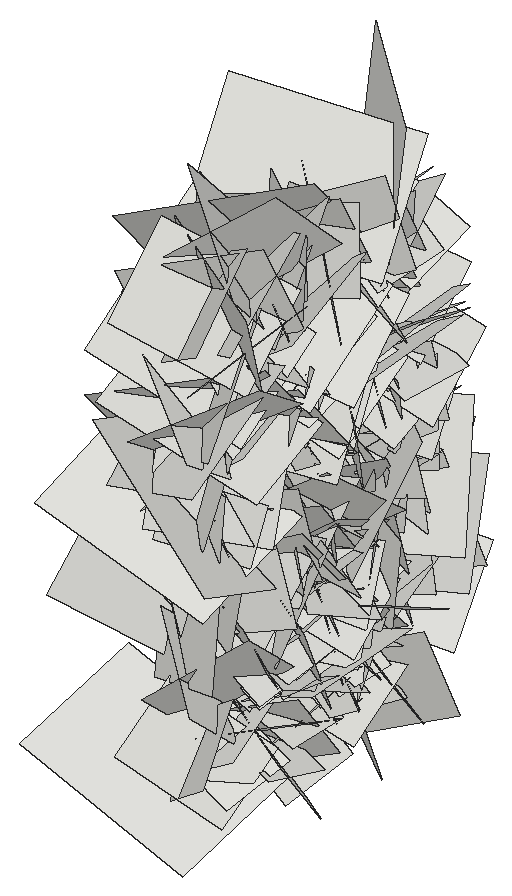
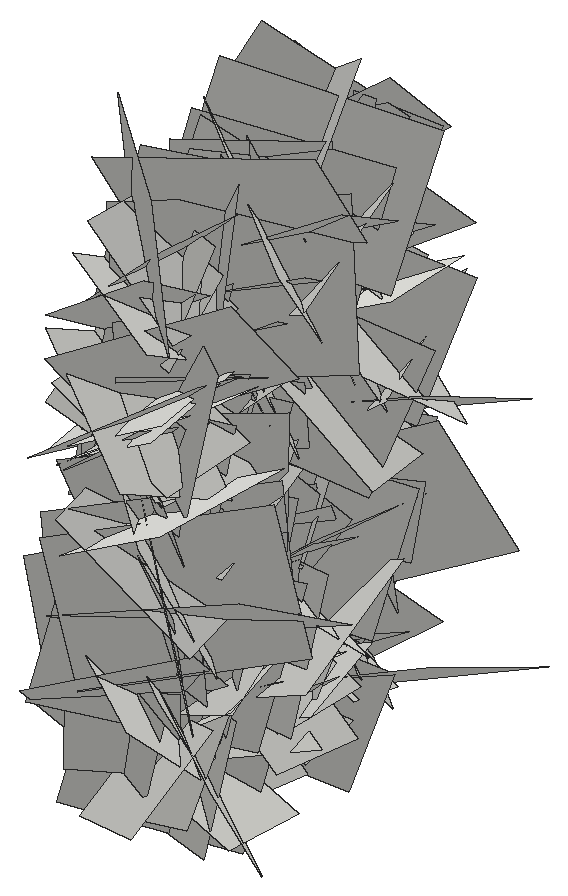
# SketchUp Ruby script. Lengths in inches.
U = 1.inch
M = Sketchup.active_model
def pt(a) = Geom::Point3d.new(a.map { |v| v * U })
def face(e, loops, mat)
  f = e.add_face(loops[0].map { |a| pt(a) })
  loops[1..].each { |l| e.add_face(l.map { |a| pt(a) }).erase! }
  f.material = f.back_material = mat if mat
  f
end
# faces: each face lists its corners as indices into pts; further lists are holes
def faces(e, pts, list, mat = nil) = list.each { |f| face(e, (f[0].is_a?(Array) ? f : [f]).map { |l| l.map { |i| pts[i] } }, mat) }
# xy, xz, yz: faces in a plane at the given z, y or x. An outline is a flat list of corners, or four numbers for a rectangle; further outlines are holes
def ring(l) = l.size == 4 ? [[l[0], l[1]], [l[2], l[1]], [l[2], l[3]], [l[0], l[3]]] : l.each_slice(2).to_a
def flat(e, list, mat, &to3) = list.each { |f| face(e, (f[0].is_a?(Array) ? f : [f]).map { |l| ring(l).map { |u, v| to3.(u, v) } }, mat) }
def xy(e, z, list, mat = nil) = flat(e, list, mat) { |x, y| [x, y, z] }
def xz(e, y, list, mat = nil) = flat(e, list, mat) { |x, z| [x, y, z] }
def yz(e, x, list, mat = nil) = flat(e, list, mat) { |y, z| [x, y, z] }
def lines(e, pts, list) = list.each { |a, b| e.add_line(pt(pts[a]), pt(pts[b])) }
# prism: a flat outline (further loops are holes) pulled along v
def prism(e, loops, v, mat = nil)
  f = face(e, loops, mat); d = Geom::Vector3d.new(v.map { |x| x * U })
  f.pushpull(f.normal.samedirection?(d) ? d.length : -d.length)
end
def box(e, o, s, mat = nil) = prism(e, [[o, [o[0] + s[0], o[1], o[2]], [o[0] + s[0], o[1] + s[1], o[2]], [o[0], o[1] + s[1], o[2]]]], [0, 0, s[2]], mat)
def at(x, y, z, deg = 0) = Geom::Transformation.translation(pt([x, y, z])) * Geom::Transformation.rotation(ORIGIN, Z_AXIS, deg.degrees)
def axes(o, x, y, z) = Geom::Transformation.new([*x, 0, *y, 0, *z, 0, *pt(o).to_a, 1])
def part(name) = M.definitions.add(name)
# library, detail: a bought-in or finely detailed component or shape, given as its bounding box
def library(name, o, s) = part(name).tap { |d| box(d.entities, o, s) }
def detail(e, o, s) = box(e.add_group.entities, o, s)
def put(e, d, t, mat = nil) = e.add_instance(d, t).tap { |i| i.material = mat if mat }
def group(e, t, mat = nil) = e.add_group.tap { |g| g.transformation = t; g.material = mat if mat }.entities
root = M.entities
c1 = part("Component\#6")
p = [[0.01,0,0],[0,3.24,4.54],[4.32,3.24,4.54],[4.33,0,0]]
faces(c1.entities,p,[[0,1,2,3]])
put(root,c1,axes([18.5,161.87,9.58],[-0.35888,-0.49511,-1.17449],[-0.11741,-1.19919,0.53746],[-1.34594,0.23663,0.26628]))
put(root,c1,axes([18.5,170.67,8.29],[-0.13658,-1.14766,-0.62909],[-0.33753,-0.58565,1.13362],[-1.34561,0.26339,-0.2205]))
put(root,c1,axes([18.5,160.65,1.35],[-0.1594,-1.22011,-0.46707],[-0.28659,-0.43091,1.2127],[-1.35486,0.2347,-0.20157]))
put(root,c1,axes([18.5,161.24,11.55],[-0.08722,-1.18104,-0.51149],[-0.30261,-0.48302,1.16122],[-1.33028,0.18731,-0.23062]))
put(root,c1,axes([18.5,161.91,24.73],[-0.20116,0.87735,-0.9177],[-0.06395,-0.93308,-0.87958],[-1.34427,-0.0869,0.17917]))
put(root,c1,axes([18.5,167.61,21.95],[-0.32344,0.31012,-1.26322],[0.1451,-1.28265,-0.34796],[-1.37111,-0.2089,0.26116]))
put(root,c1,axes([18.5,171.01,11.29],[-0.23144,-0.15428,-1.27652],[0.01824,-1.29503,0.15357],[-1.36284,0.00887,0.21884]))
put(root,c1,axes([18.5,161.07,7.88],[-0.0926,0.91308,0.78861],[-0.24837,0.76278,-0.90913],[-1.25453,-0.21841,0.12178]))
put(root,c1,axes([18.5,170.58,10.37],[-0.24309,-1.14649,0.14454],[-0.04952,0.15643,1.16674],[-1.2239,0.22139,-0.07591]))
put(root,c1,axes([18.5,165.1,2.71],[0.06092,-1.21711,0.58199],[-0.18306,0.57109,1.21136],[-1.41828,-0.12599,-0.13136]))
put(root,c1,axes([18.5,162.31,11.53],[-0.17206,0.75955,-0.87532],[-0.12131,-0.89005,-0.75111],[-1.22246,-0.01858,0.19774]))
put(root,c1,axes([18.5,157.93,15.34],[-0.27083,1.19165,0.15594],[0.0802,0.17506,-1.21378],[-1.27139,-0.2428,-0.10978]))
put(root,c1,axes([18.5,168.375,23.9],[0.0952,-0.72561,-1.04974],[-0.29336,-1.03837,0.69407],[-1.32049,0.17837,-0.22987]))
put(root,c1,axes([18.5,159.14,18.38],[-0.07521,0.79304,-0.86536],[-0.12573,-0.86735,-0.78513],[-1.23784,0.03991,0.13233]))
put(root,c1,axes([18.5,155.03,14.95],[0.10989,1.07322,0.82249],[-0.07177,0.82799,-1.07186],[-1.43147,0.04087,0.11688]))
put(root,c1,axes([18.5,166.4,18.65],[0.092,-1.19571,-0.63762],[-0.0325,-0.6405,1.19693],[-1.43603,-0.06211,-0.06794]))
put(root,c1,axes([18.5,159.69,18.96],[-0.02704,0.74145,1.09535],[0.09362,1.09406,-0.73853],[-1.39894,0.05888,-0.07059]))
put(root,c1,axes([18.5,163.36,23.49],[-0.04873,0.57368,-1.00395],[-0.12423,-1.00188,-0.56714],[-1.21936,0.07915,0.09791]))
put(root,c1,axes([18.5,162.85,15.75],[-0.04254,-1.00522,0.67204],[-0.02385,0.67292,1.00519],[-1.28151,0.02084,-0.04102]))
put(root,c1,axes([18.5,163.86,1.73],[-0.03729,0.66749,1.03354],[0.00972,1.03407,-0.66752],[-1.30413,-0.01138,-0.03452]))
put(root,c1,axes([18.5,161.03,16.77],[0.02327,0.73455,-0.90907],[-0.17416,-0.89826,-0.72978],[-1.22657,0.14148,0.08637]))
put(root,c1,axes([18.5,162.03,18.62],[-0.15865,-0.78055,-0.79386],[0.03617,-0.80384,0.78393],[-1.17956,0.08034,0.13081]))
put(root,c1,axes([18.5,161.02,12.77],[-0.04866,0.36936,-1.04237],[-0.12613,-1.03886,-0.36288],[-1.16543,0.09701,0.0828]))
put(root,c1,axes([18.5,163.21,2.24],[0.08398,-0.53221,1.10764],[-0.11648,1.10243,0.53756],[-1.29738,-0.13342,0.02343]))
put(root,c1,axes([18.5,155.93,16.01],[-0.06166,0.77521,1.08886],[0.24821,1.07895,-0.75564],[-1.39492,0.15772,-0.18259]))
put(root,c1,axes([14.53,164.09,3.1],[-0.16189,-0.51758,0.36968],[-0.06161,0.38995,0.52196],[0.67139,-0.08902,0.13704]))
put(root,c1,axes([18.5,165.97,13.03],[-0.11695,-0.23373,1.15092],[0.10796,1.14973,0.24325],[-1.24018,0.12213,-0.08736]))
put(root,c1,axes([18.5,170.79,17.67],[-0.07972,-0.69903,-0.88266],[0.01234,-0.88506,0.69994],[-1.19343,0.03754,0.0662]))
put(root,c1,axes([18.5,164.53,2.65],[-0.11418,0.95876,0.15487],[-0.16789,0.13639,-0.95453],[-1.01568,-0.13033,0.14037]))
put(root,c1,axes([18.5,165.6875,8.33],[-0.14254,-0.77018,0.64298],[-0.05856,0.65343,0.77114],[-1.06187,0.06735,-0.12884]))
put(root,c1,axes([14.53,159.77,13.93],[-0.14822,0.47929,0.38572],[0.01533,0.39801,-0.48932],[0.65196,0.0996,0.0992]))
put(root,c1,axes([18.5,164.18,5.53],[-0.00871,-1.21515,-0.1589],[0.11926,-0.15898,1.20995],[-1.29354,-0.00648,0.11262]))
put(root,c1,axes([18.5,168.99,0.33],[-0.20008,-0.71049,0.66963],[0.07161,0.67089,0.73087],[-1.03242,0.18422,-0.07908]))
put(root,c1,axes([18.5,166.625,12.7],[-0.17127,1.04033,-0.10676],[0.13463,-0.08771,-1.04688],[-1.10034,-0.17266,-0.11147]))
put(root,c1,axes([18.5,160.14,4.78],[-0.03826,-0.47304,0.81506],[-0.18962,0.80427,0.45886],[-0.98077,-0.13704,-0.12051]))
put(root,c1,axes([14.53,170.02,6.34],[-0.13634,-0.30577,-0.6303],[-0.02329,-0.63876,0.31436],[0.74222,-0.07621,-0.10592]))
put(root,c1,axes([18.5,156.14,6.5],[-0.17845,0.35117,0.84391],[-0.01887,0.85668,-0.36003],[-0.96872,-0.08137,-0.14844]))
put(root,c1,axes([18.5,163.93,5.47],[-0.11462,-1.01834,-0.26907],[0.10191,-0.2789,1.0169],[-1.11183,0.07941,0.12095]))
put(root,c1,axes([14.53,162.91,7.6875],[-0.03517,0.6334,0.29771],[-0.1292,0.28826,-0.62688],[0.73053,0.08147,-0.09654]))
put(root,c1,axes([18.5,160.62,5.12],[-0.08568,1.04485,0.18773],[0.09569,0.19436,-1.04286],[-1.1212,-0.06325,-0.10335]))
put(root,c1,axes([18.5,162.44,14.8125],[0.22172,-1.13603,-0.19278],[-0.19013,-0.22565,1.13507],[-1.20652,-0.17321,-0.21429]))
put(root,c1,axes([18.5,159.91,9.22],[0.2022,-1.20502,0.50539],[0.1049,0.52261,1.20871],[-1.38114,-0.13672,0.1658]))
put(root,c1,axes([18.5,163.57,3.71],[-0.11292,-0.2033,0.99476],[0.09749,0.99417,0.21302],[-1.07181,0.11185,-0.08542]))
put(root,c1,axes([18.5,166.01,11.8],[-0.21466,0.53877,-0.68228],[0.03009,-0.69607,-0.55809],[-0.92102,-0.14831,0.14079]))
put(root,c1,axes([18.5,168.87,14.79],[-0.03205,0.06087,-1.12787],[0.16204,-1.11767,-0.06442],[-1.18627,-0.15431,0.02167]))
put(root,c1,axes([18.5,167.18,1.59],[0.07507,-1.0991,0.32301],[0.05871,0.32653,1.09895],[-1.2129,-0.05222,0.07319]))
put(root,c1,axes([18.5,157.18,19.73],[0.07599,0.81527,0.8297],[0.084,0.82592,-0.8184],[-1.23014,0.10676,-0.00463]))
put(root,c1,axes([18.5,167.28,17.92],[0.19972,-0.96368,-0.57877],[-0.14667,-0.60226,0.95775],[-1.18251,-0.08806,-0.21655]))
put(root,c1,axes([18.5,167.22,15.375],[0.0235,-0.92066,-0.53568],[0.01768,-0.53543,0.92093],[-1.12894,-0.02755,0.00327]))
put(root,c1,axes([14.53,162.79,15.86],[-0.07285,0.46729,0.4905],[0.02436,0.49435,-0.46773],[0.71769,0.03066,0.06566]))
put(root,c1,axes([14.53,161.25,17.66],[-0.25985,0.898,-0.37026],[-0.14737,-0.41038,-0.90325],[1.01902,0.16964,-0.22504]))
put(root,c1,axes([14.53,165.96,10.85],[-0.09912,0.20412,-0.70693],[-0.02587,-0.71308,-0.20267],[0.77953,0.00229,-0.09661]))
put(root,c1,axes([18.5,169.19,10.7],[0.0913,0.46499,-1.24639],[0.29576,-1.22753,-0.43867],[-1.37875,-0.23253,-0.17663]))
put(root,c1,axes([18.5,168.14,0.12],[0.06773,-0.63363,0.78179],[-0.11595,0.77435,0.63654],[-1.06038,-0.12515,-0.01967]))
put(root,c1,axes([18.5,166.18,19.56],[0.12535,0.0531,1.28965],[0.2192,1.27754,-0.07157],[-1.35051,0.21229,0.10808]))
put(root,c1,axes([18.5,167.01,8.33],[-0.18631,0.3359,0.73427],[-0.04897,0.74605,-0.35235],[-0.8545,-0.11599,-0.1399]))
put(root,c1,axes([14.53,159.82,10.86],[-0.164,0.05549,-0.7166],[0.119,-0.72215,-0.08015],[0.75252,0.12629,-0.14349]))
put(root,c1,axes([18.5,164.72,6.23],[0.02586,0.29335,1.1723],[0.23754,1.1511,-0.29271],[-1.25874,0.22326,-0.03115]))
put(root,c1,axes([14.53,164.71,11.17],[-0.09162,-0.23701,0.75882],[-0.09076,0.76162,0.22813],[0.83777,0.05659,0.1077]))
put(root,c1,axes([14.53,167.39,12.19],[-0.06725,0.11282,-0.6237],[0.12717,-0.61335,-0.12315],[0.65971,0.12973,-0.03984]))
put(root,c1,axes([14.53,158.25,7.85],[0.01053,0.60228,-0.51533],[-0.19634,-0.49934,-0.58716],[0.81696,-0.12777,-0.13447]))
put(root,c1,axes([18.5,165.51,17.74],[-0.00528,-0.97827,-0.44464],[0.11526,-0.44282,0.97306],[-1.13321,-0.04048,0.10104]))
put(root,c1,axes([18.5,165.75,-1.09],[0.03685,-0.4153,0.96157],[0.02645,0.96216,0.41465],[-1.10996,0.00914,0.04181]))
put(root,c1,axes([18.5,167.74,3.51],[0.11337,-0.86322,0.3774],[-0.28126,0.33685,0.84566],[-0.95821,-0.201,-0.20357]))
put(root,c1,axes([18.5,161.03,4.22],[-0.00206,0.54706,-0.73945],[-0.10036,-0.73565,-0.544],[-0.96983,0.07497,0.05787]))
put(root,c1,axes([18.5,158.84,13.7],[-0.15038,-0.75335,0.50607],[0.08727,0.49942,0.76653],[-0.95804,0.16374,-0.00961]))
put(root,c1,axes([18.5,166.72,20.27],[-0.14718,0.45385,-0.66356],[-0.05291,-0.67695,-0.45256],[-0.85051,-0.03642,0.14299]))
put(root,c1,axes([14.53,158.82,19.64],[0.09205,0.73549,-0.019],[-0.17536,0.00088,-0.72213],[0.75991,-0.08889,-0.16434]))
put(root,c1,axes([18.5,169.09,13.37],[-0.12805,-0.81492,0.2825],[0.01832,0.28292,0.8235],[-0.91406,0.11983,-0.02307]))
put(root,c1,axes([14.53,159.61,12.59],[0.0897,0.16152,-0.57424],[0.01993,-0.58042,-0.16049],[0.632,-0.00462,0.08656]))
put(root,c1,axes([14.53,160.65,18.69],[0.1336,-0.1743,0.59472],[-0.06624,0.60023,0.18916],[0.65357,0.09646,-0.1024]))
put(root,c1,axes([14.53,160.54,14.42],[-0.065,-0.29459,-0.75204],[-0.0763,-0.74921,0.29935],[0.85274,-0.0895,-0.03054]))
put(root,c1,axes([14.53,161.26,10.83],[-0.08958,0.45503,-0.59155],[0.06652,-0.58889,-0.46195],[0.78829,0.10141,-0.02824]))
put(root,c1,axes([18.5,170.16,13.55],[0.14984,-1.04824,-0.22204],[-0.00627,-0.22472,1.05715],[-1.13577,-0.13705,-0.03513]))
put(root,c1,axes([14.53,160.97,6.7],[0.04912,0.73058,0.10133],[-0.09877,0.10652,-0.72536],[0.77557,-0.03271,-0.0988]))
put(root,c1,axes([18.5,163.26,10.51],[-0.09772,0.8385,-0.3881],[0.10419,-0.37892,-0.842],[-0.97385,-0.12468,-0.05114]))
put(root,c1,axes([14.53,159.79,25.07],[-0.1328,0.69586,-0.68383],[-0.18687,-0.69425,-0.67416],[1.01714,-0.03669,-0.21313]))
put(root,c1,axes([18.5,167.39,3.05],[0.22625,-1.02118,-0.283],[-0.12014,-0.30902,1.02962],[-1.11681,-0.17363,-0.16809]))
put(root,c1,axes([14.53,159.32,12.84],[0.06752,-0.16321,-0.59207],[0.0871,-0.58763,0.17083],[0.64514,0.09641,0.0389]))
put(root,c1,axes([14.53,169.73,5.36],[0.07377,0.11031,-0.61615],[0.06228,-0.61836,-0.10407],[0.66058,0.04598,0.07863]))
put(root,c1,axes([18.5,166.22,16.78],[0.0558,0.90138,-0.08554],[-0.09664,-0.07998,-0.89882],[-0.95488,0.06076,0.08597]))
put(root,c1,axes([14.53,166.8,6.58],[-0.19077,-0.84984,-0.315],[0.00737,-0.32244,0.86593],[0.9607,-0.16629,-0.0692]))
put(root,c1,axes([18.5,159.03,23.29],[0.13252,0.38295,-0.87838],[-0.10893,-0.87536,-0.39626],[-1.00987,0.14467,-0.07253]))
put(root,c1,axes([14.53,160.57,3.12],[0.03509,0.82869,0.13415],[-0.15764,0.13792,-0.81528],[0.87577,-0.00838,-0.15213]))
put(root,c1,axes([14.53,164.04,15.7],[0.03624,-0.6234,-0.24842],[0.08,-0.24359,0.62167],[0.70683,0.05954,-0.05762]))
put(root,c1,axes([18.5,170.98,12.21],[0.31631,-0.51758,-1.19288],[0.16648,-1.20059,0.56021],[-1.36826,-0.26573,-0.20761]))
put(root,c1,axes([14.53,169.83,13.22],[0.13817,-0.64015,-0.16037],[-0.03989,-0.17041,0.64965],[0.69839,0.11692,0.06883]))
put(root,c1,axes([14.53,161.46,7.67],[0.11157,-0.00104,0.59962],[0.09459,0.60203,-0.01462],[0.62852,-0.09042,-0.10424]))
put(root,c1,axes([18.5,168.08,9.41],[0.11593,0.02752,-0.90523],[-0.14705,-0.90054,-0.04413],[-0.94866,0.14295,-0.10378]))
put(root,c1,axes([14.53,169.26,18.83],[0.02849,-0.83115,-0.05333],[-0.13283,-0.05679,0.82186],[0.87278,0.01849,0.12683]))
put(root,c1,axes([14.53,165.55,15.88],[-0.02597,-0.35934,-0.67832],[0.02345,-0.67872,0.35875],[0.81334,0.00809,-0.032]))
put(root,c1,axes([14.53,167.12,21.5],[0.0656,0.35319,-0.61189],[0.00255,-0.61434,-0.35436],[0.7489,-0.02885,0.0548]))
put(root,c1,axes([18.5,164.04,2.37],[0.08884,-0.86849,0.07962],[-0.14736,0.06566,0.86256],[-0.91264,-0.09515,-0.13152]))
put(root,c1,axes([18.5,162.54,0.74],[0.05881,-0.79857,0.25436],[-0.14334,0.24305,0.79255],[-0.87675,-0.0933,-0.11251]))
put(root,c1,axes([18.5,157.37,3.29],[-0.12325,0.67494,0.21472],[-0.06797,0.20667,-0.68436],[-0.74769,-0.13004,0.02682]))
put(root,c1,axes([18.5,166.02,4.84],[0.16866,0.71959,0.68076],[-0.0323,0.69272,-0.72511],[-1.04952,0.09433,0.13172]))
put(root,c1,axes([14.53,162.4,12.14],[0.15913,-0.1111,0.71617],[-0.10617,0.72117,0.13287],[0.76084,0.12387,-0.13124]))
put(root,c1,axes([14.53,165.06,16.01],[-0.24936,0.99659,0.4051],[-0.07669,0.39908,-1.02378],[1.13774,0.24532,0.01978]))
put(root,c1,axes([14.53,164.7,6.68],[-0.19863,-0.78204,0.62344],[-0.03401,0.63866,0.7915],[1.0596,-0.1261,0.14227]))
put(root,c1,axes([18.5,166.67,11.65],[-0.03639,0.32382,0.70516],[-0.0632,0.70266,-0.32558],[-0.82009,-0.06852,-0.0062]))
put(root,c1,axes([18.5,166.25,3.34],[-0.10377,-0.78092,-0.09398],[0.04515,-0.09983,0.78516],[-0.83253,0.09192,0.05429]))
put(root,c1,axes([18.5,167.84,10.46],[0.01526,0.23241,-0.73689],[-0.14958,-0.72384,-0.23105],[-0.80526,0.13886,0.02896]))
put(root,c1,axes([18.5,164.66,7.18],[0.03191,0.54978,-0.59147],[-0.106,-0.58478,-0.54866],[-0.84939,0.09364,0.04625]))
put(root,c1,axes([18.5,155.24,20.59],[-0.01301,0.69003,0.71111],[0.211,0.69839,-0.67424],[-1.02891,0.13449,-0.14726]))
put(root,c1,axes([18.5,167.39,19.82],[-0.12929,0.6108,0.35138],[-0.02449,0.35295,-0.62154],[-0.74654,-0.11736,-0.04046]))
put(root,c1,axes([14.53,165.07,9.38],[0.13081,0.27606,-0.70722],[-0.08788,-0.70731,-0.29057],[0.79993,-0.12284,0.08373]))
put(root,c1,axes([18.5,159.79,6],[0.13547,0.51146,0.93772],[0.15367,0.92736,-0.52557],[-1.12174,0.18881,0.04125]))
put(root,c1,axes([18.5,159.9,13.67],[0.02397,0.44215,0.82689],[0.11898,0.8199,-0.44149],[-0.98679,0.1096,-0.03314]))
put(root,c1,axes([14.53,164.44,22.83],[-0.02931,-0.02413,-0.88007],[-0.04764,-0.87932,0.02552],[0.93201,-0.0457,-0.02637]))
put(root,c1,axes([18.5,168.54,15.47],[0.051,0.16682,-0.79913],[-0.09039,-0.79511,-0.17112],[-0.86061,0.0934,-0.02938]))
put(root,c1,axes([18.5,155.625,2.89],[-0.13104,0.56412,0.5606],[0.11872,0.57403,-0.55293],[-0.83462,-0.00692,-0.16667]))
put(root,c1,axes([18.5,163.43,17.5],[0.07736,-0.30856,0.98844],[0.18729,0.98007,0.2929],[-1.08152,0.14765,0.12143]))
put(root,c1,axes([14.53,163.43,17.5],[-0.07736,-0.30856,0.98844],[-0.18729,0.98007,0.2929],[1.08152,0.14765,0.12143]))
put(root,c1,axes([14.53,155.625,2.89],[0.13104,0.56412,0.5606],[-0.11872,0.57403,-0.55293],[0.83462,-0.00692,-0.16667]))
put(root,c1,axes([14.53,168.54,15.47],[-0.051,0.16682,-0.79913],[0.09039,-0.79511,-0.17112],[0.86061,0.0934,-0.02938]))
put(root,c1,axes([18.5,164.44,22.83],[0.02931,-0.02413,-0.88007],[0.04764,-0.87932,0.02552],[-0.93201,-0.0457,-0.02637]))
put(root,c1,axes([14.53,159.9,13.67],[-0.02397,0.44215,0.82689],[-0.11898,0.8199,-0.44149],[0.98679,0.1096,-0.03314]))
put(root,c1,axes([14.53,159.79,6],[-0.13547,0.51146,0.93772],[-0.15367,0.92736,-0.52557],[1.12174,0.18881,0.04125]))
put(root,c1,axes([18.5,165.07,9.38],[-0.13081,0.27606,-0.70722],[0.08788,-0.70731,-0.29057],[-0.79993,-0.12284,0.08373]))
put(root,c1,axes([14.53,167.39,19.82],[0.12929,0.6108,0.35138],[0.02449,0.35295,-0.62154],[0.74654,-0.11736,-0.04046]))
put(root,c1,axes([14.53,155.24,20.59],[0.01301,0.69003,0.71111],[-0.211,0.69839,-0.67424],[1.02891,0.13449,-0.14726]))
put(root,c1,axes([14.53,164.66,7.18],[-0.03191,0.54978,-0.59147],[0.106,-0.58478,-0.54866],[0.84939,0.09364,0.04625]))
put(root,c1,axes([14.53,167.84,10.46],[-0.01526,0.23241,-0.73689],[0.14958,-0.72384,-0.23105],[0.80526,0.13886,0.02896]))
put(root,c1,axes([14.53,166.25,3.34],[0.10377,-0.78092,-0.09398],[-0.04515,-0.09983,0.78516],[0.83253,0.09192,0.05429]))
put(root,c1,axes([14.53,166.67,11.65],[0.03639,0.32382,0.70516],[0.0632,0.70266,-0.32558],[0.82009,-0.06852,-0.0062]))
put(root,c1,axes([18.5,164.7,6.68],[0.19863,-0.78204,0.62344],[0.03401,0.63866,0.7915],[-1.0596,-0.1261,0.14227]))
put(root,c1,axes([18.5,165.06,16.01],[0.24936,0.99659,0.4051],[0.07669,0.39908,-1.02378],[-1.13774,0.24532,0.01978]))
put(root,c1,axes([18.5,162.4,12.14],[-0.15913,-0.1111,0.71617],[0.10617,0.72117,0.13287],[-0.76084,0.12387,-0.13124]))
put(root,c1,axes([14.53,166.02,4.84],[-0.16866,0.71959,0.68076],[0.0323,0.69272,-0.72511],[1.04952,0.09433,0.13172]))
put(root,c1,axes([14.53,157.37,3.29],[0.12325,0.67494,0.21472],[0.06797,0.20667,-0.68436],[0.74769,-0.13004,0.02682]))
put(root,c1,axes([14.53,162.54,0.74],[-0.05881,-0.79857,0.25436],[0.14334,0.24305,0.79255],[0.87675,-0.0933,-0.11251]))
put(root,c1,axes([14.53,164.04,2.37],[-0.08884,-0.86849,0.07962],[0.14736,0.06566,0.86256],[0.91264,-0.09515,-0.13152]))
put(root,c1,axes([18.5,167.12,21.5],[-0.0656,0.35319,-0.61189],[-0.00255,-0.61434,-0.35436],[-0.7489,-0.02885,0.0548]))
put(root,c1,axes([18.5,165.55,15.88],[0.02597,-0.35934,-0.67832],[-0.02345,-0.67872,0.35875],[-0.81334,0.00809,-0.032]))
put(root,c1,axes([18.5,169.26,18.83],[-0.02849,-0.83115,-0.05333],[0.13283,-0.05679,0.82186],[-0.87278,0.01849,0.12683]))
put(root,c1,axes([14.53,168.08,9.41],[-0.11593,0.02752,-0.90523],[0.14705,-0.90054,-0.04413],[0.94866,0.14295,-0.10378]))
put(root,c1,axes([18.5,161.46,7.67],[-0.11157,-0.00104,0.59962],[-0.09459,0.60203,-0.01462],[-0.62852,-0.09042,-0.10424]))
put(root,c1,axes([18.5,169.83,13.22],[-0.13817,-0.64015,-0.16037],[0.03989,-0.17041,0.64965],[-0.69839,0.11692,0.06883]))
put(root,c1,axes([14.53,170.98,12.21],[-0.31631,-0.51758,-1.19288],[-0.16648,-1.20059,0.56021],[1.36826,-0.26573,-0.20761]))
put(root,c1,axes([18.5,164.04,15.7],[-0.03624,-0.6234,-0.24842],[-0.08,-0.24359,0.62167],[-0.70683,0.05954,-0.05762]))
put(root,c1,axes([18.5,160.57,3.12],[-0.03509,0.82869,0.13415],[0.15764,0.13792,-0.81528],[-0.87577,-0.00838,-0.15213]))
put(root,c1,axes([14.53,159.03,23.29],[-0.13252,0.38295,-0.87838],[0.10893,-0.87536,-0.39626],[1.00987,0.14467,-0.07253]))
put(root,c1,axes([18.5,166.8,6.58],[0.19077,-0.84984,-0.315],[-0.00737,-0.32244,0.86593],[-0.9607,-0.16629,-0.0692]))
put(root,c1,axes([14.53,166.22,16.78],[-0.0558,0.90138,-0.08554],[0.09664,-0.07998,-0.89882],[0.95488,0.06076,0.08597]))
put(root,c1,axes([18.5,169.73,5.36],[-0.07377,0.11031,-0.61615],[-0.06228,-0.61836,-0.10407],[-0.66058,0.04598,0.07863]))
put(root,c1,axes([18.5,159.32,12.84],[-0.06752,-0.16321,-0.59207],[-0.0871,-0.58763,0.17083],[-0.64514,0.09641,0.0389]))
put(root,c1,axes([14.53,167.39,3.05],[-0.22625,-1.02118,-0.283],[0.12014,-0.30902,1.02962],[1.11681,-0.17363,-0.16809]))
put(root,c1,axes([18.5,159.79,25.07],[0.1328,0.69586,-0.68383],[0.18687,-0.69425,-0.67416],[-1.01714,-0.03669,-0.21313]))
put(root,c1,axes([14.53,163.26,10.51],[0.09772,0.8385,-0.3881],[-0.10419,-0.37892,-0.842],[0.97385,-0.12468,-0.05114]))
put(root,c1,axes([18.5,160.97,6.7],[-0.04912,0.73058,0.10133],[0.09877,0.10652,-0.72536],[-0.77557,-0.03271,-0.0988]))
put(root,c1,axes([14.53,170.16,13.55],[-0.14984,-1.04824,-0.22204],[0.00627,-0.22472,1.05715],[1.13577,-0.13705,-0.03513]))
put(root,c1,axes([18.5,161.26,10.83],[0.08958,0.45503,-0.59155],[-0.06652,-0.58889,-0.46195],[-0.78829,0.10141,-0.02824]))
put(root,c1,axes([18.5,160.54,14.42],[0.065,-0.29459,-0.75204],[0.0763,-0.74921,0.29935],[-0.85274,-0.0895,-0.03054]))
put(root,c1,axes([18.5,160.65,18.69],[-0.1336,-0.1743,0.59472],[0.06624,0.60023,0.18916],[-0.65357,0.09646,-0.1024]))
put(root,c1,axes([18.5,159.61,12.59],[-0.0897,0.16152,-0.57424],[-0.01993,-0.58042,-0.16049],[-0.632,-0.00462,0.08656]))
put(root,c1,axes([14.53,169.09,13.37],[0.12805,-0.81492,0.2825],[-0.01832,0.28292,0.8235],[0.91406,0.11983,-0.02307]))
put(root,c1,axes([18.5,158.82,19.64],[-0.09205,0.73549,-0.019],[0.17536,0.00088,-0.72213],[-0.75991,-0.08889,-0.16434]))
put(root,c1,axes([14.53,166.72,20.27],[0.14718,0.45385,-0.66356],[0.05291,-0.67695,-0.45256],[0.85051,-0.03642,0.14299]))
put(root,c1,axes([14.53,158.84,13.7],[0.15038,-0.75335,0.50607],[-0.08727,0.49942,0.76653],[0.95804,0.16374,-0.00961]))
put(root,c1,axes([14.53,161.03,4.22],[0.00206,0.54706,-0.73945],[0.10036,-0.73565,-0.544],[0.96983,0.07497,0.05787]))
put(root,c1,axes([14.53,167.74,3.51],[-0.11337,-0.86322,0.3774],[0.28126,0.33685,0.84566],[0.95821,-0.201,-0.20357]))
put(root,c1,axes([14.53,165.75,-1.09],[-0.03685,-0.4153,0.96157],[-0.02645,0.96216,0.41465],[1.10996,0.00914,0.04181]))
put(root,c1,axes([14.53,165.51,17.74],[0.00528,-0.97827,-0.44464],[-0.11526,-0.44282,0.97306],[1.13321,-0.04048,0.10104]))
put(root,c1,axes([18.5,158.25,7.85],[-0.01053,0.60228,-0.51533],[0.19634,-0.49934,-0.58716],[-0.81696,-0.12777,-0.13447]))
put(root,c1,axes([18.5,167.39,12.19],[0.06725,0.11282,-0.6237],[-0.12717,-0.61335,-0.12315],[-0.65971,0.12973,-0.03984]))
put(root,c1,axes([18.5,164.71,11.17],[0.09162,-0.23701,0.75882],[0.09076,0.76162,0.22813],[-0.83777,0.05659,0.1077]))
put(root,c1,axes([14.53,164.72,6.23],[-0.02586,0.29335,1.1723],[-0.23754,1.1511,-0.29271],[1.25874,0.22326,-0.03115]))
put(root,c1,axes([18.5,159.82,10.86],[0.164,0.05549,-0.7166],[-0.119,-0.72215,-0.08015],[-0.75252,0.12629,-0.14349]))
